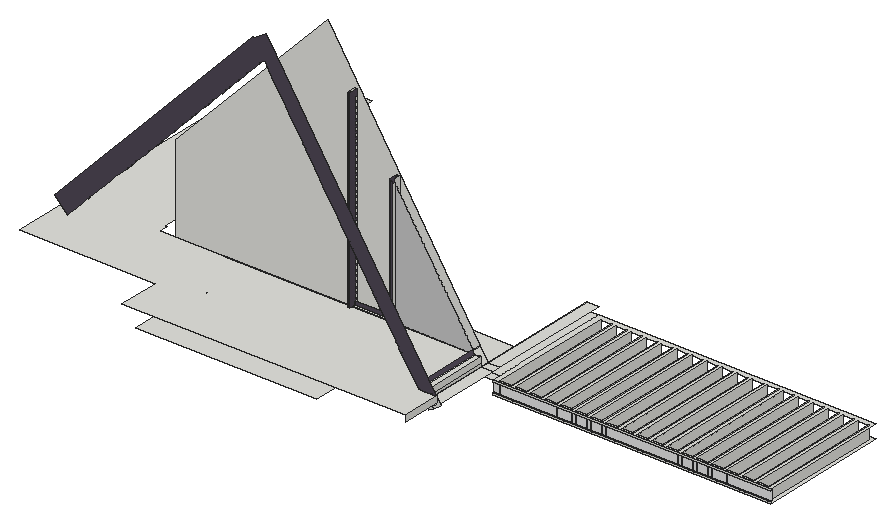
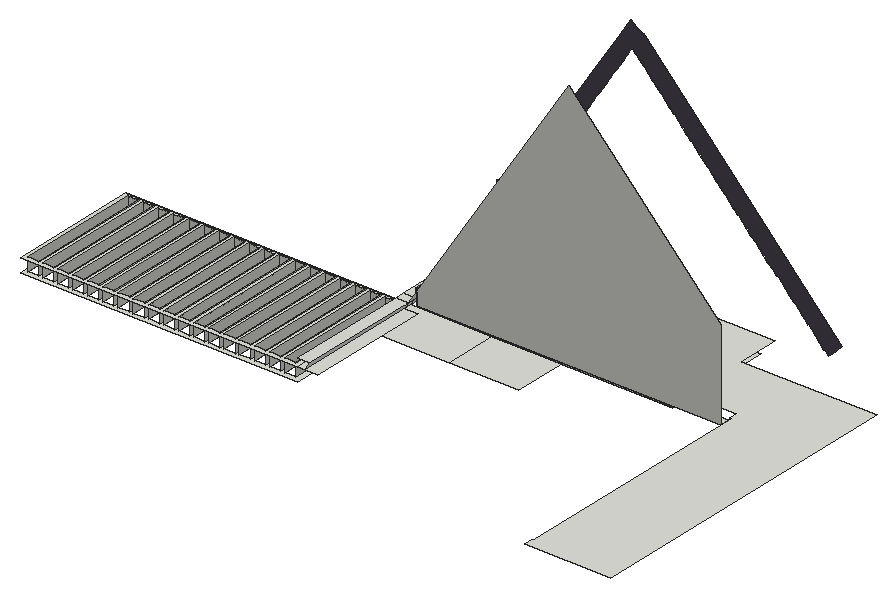
# SketchUp Ruby script. Lengths in inches.
U = 1.inch
M = Sketchup.active_model
def pt(a) = Geom::Point3d.new(a.map { |v| v * U })
def face(e, loops, mat)
  f = e.add_face(loops[0].map { |a| pt(a) })
  loops[1..].each { |l| e.add_face(l.map { |a| pt(a) }).erase! }
  f.material = f.back_material = mat if mat
  f
end
# faces: each face lists its corners as indices into pts; further lists are holes
def faces(e, pts, list, mat = nil) = list.each { |f| face(e, (f[0].is_a?(Array) ? f : [f]).map { |l| l.map { |i| pts[i] } }, mat) }
# xy, xz, yz: faces in a plane at the given z, y or x. An outline is a flat list of corners, or four numbers for a rectangle; further outlines are holes
def ring(l) = l.size == 4 ? [[l[0], l[1]], [l[2], l[1]], [l[2], l[3]], [l[0], l[3]]] : l.each_slice(2).to_a
def flat(e, list, mat, &to3) = list.each { |f| face(e, (f[0].is_a?(Array) ? f : [f]).map { |l| ring(l).map { |u, v| to3.(u, v) } }, mat) }
def xy(e, z, list, mat = nil) = flat(e, list, mat) { |x, y| [x, y, z] }
def xz(e, y, list, mat = nil) = flat(e, list, mat) { |x, z| [x, y, z] }
def yz(e, x, list, mat = nil) = flat(e, list, mat) { |y, z| [x, y, z] }
def lines(e, pts, list) = list.each { |a, b| e.add_line(pt(pts[a]), pt(pts[b])) }
# prism: a flat outline (further loops are holes) pulled along v
def prism(e, loops, v, mat = nil)
  f = face(e, loops, mat); d = Geom::Vector3d.new(v.map { |x| x * U })
  f.pushpull(f.normal.samedirection?(d) ? d.length : -d.length)
end
def box(e, o, s, mat = nil) = prism(e, [[o, [o[0] + s[0], o[1], o[2]], [o[0] + s[0], o[1] + s[1], o[2]], [o[0], o[1] + s[1], o[2]]]], [0, 0, s[2]], mat)
def at(x, y, z, deg = 0) = Geom::Transformation.translation(pt([x, y, z])) * Geom::Transformation.rotation(ORIGIN, Z_AXIS, deg.degrees)
def axes(o, x, y, z) = Geom::Transformation.new([*x, 0, *y, 0, *z, 0, *pt(o).to_a, 1])
def part(name) = M.definitions.add(name)
# library, detail: a bought-in or finely detailed component or shape, given as its bounding box
def library(name, o, s) = part(name).tap { |d| box(d.entities, o, s) }
def detail(e, o, s) = box(e.add_group.entities, o, s)
def put(e, d, t, mat = nil) = e.add_instance(d, t).tap { |i| i.material = mat if mat }
def group(e, t, mat = nil) = e.add_group.tap { |g| g.transformation = t; g.material = mat if mat }.entities
root = M.entities
M.materials.add("[Color M01]").color = [226, 226, 226]
M.materials.add("[Color M02]").color = [198, 198, 198]
M.materials.add("[Color M06]").color = [79, 71, 84]
c1 = library("A$C06767DEF\#1",[-8.3,1.21,0],[7.09,7.09,5.51])
xy(root,240.88,[[[2459.77,521.5625,2674.15,623.84],[2662.75,523.31,2671.43,620.37],[2651.06,523.31,2659.75,620.37],[2639.37,523.31,2648.06,620.37],[2627.68,523.31,2636.37,620.37],[2616,523.31,2624.68,620.37],[2604.31,523.31,2613,620.37],[2592.62,523.31,2601.31,620.37],[2580.93,523.31,2589.62,620.37],[2569.25,523.31,2577.93,620.37],[2557.56,523.31,2566.25,620.37],[2545.87,523.31,2554.56,620.37],[2534.18,523.31,2542.87,620.37],[2522.5,523.31,2531.18,620.37],[2510.81,523.31,2519.5,620.37],[2499.12,523.31,2507.81,620.37],[2487.43,523.31,2496.12,620.37],[2475.75,523.31,2484.43,620.37],[2464.06,523.31,2472.75,620.37]]])
xy(root,242.34,[[2459.77,521.5625,2674.15,522.8125]])
xy(root,249.61,[[2459.77,521.5625,2674.15,522.8125]])
xy(root,250.875,[[[2251.48,437.0625,2251.48,509.6875,2337.96,509.6875,2337.96,521.5625,2391.36,521.5625,2391.36,437.0625],[2357.39,456.39,2358.94,456.6,2360.39,457.2,2361.63,458.15,2362.59,459.39,2363.1875,460.84,2363.39,462.39,2363.1875,463.95,2362.59,465.39,2361.63,466.64,2360.39,467.59,2358.94,468.1875,2357.39,468.39,2355.84,468.1875,2354.39,467.59,2353.15,466.64,2352.19,465.39,2351.59,463.95,2351.39,462.39,2351.59,460.84,2352.19,459.39,2353.15,458.15,2354.39,457.2,2355.84,456.6],[2294.3125,459.39,2295.87,459.6,2297.3125,460.2,2298.56,461.15,2299.51,462.39,2300.11,463.84,2300.3125,465.39,2300.11,466.95,2299.51,468.39,2298.56,469.64,2297.3125,470.59,2295.87,471.1875,2294.3125,471.39,2292.76,471.1875,2291.3125,470.59,2290.07,469.64,2289.12,468.39,2288.52,466.95,2288.3125,465.39,2288.52,463.84,2289.12,462.39,2290.07,461.15,2291.3125,460.2,2292.76,459.6]]])
xy(root,251.0625,[[2251.48,509.6875,2337.96,521.5625],[2337.96,521.5625,2391.36,562.32],[2391.36,521.5625,2391.36,562.32,2444.26,562.32,2444.26,527.76,2459.77,527.76,2459.77,521.5625],[[2459.77,521.5625,2674.15,623.84],[2662.75,523.31,2671.43,620.37],[2651.06,523.31,2659.75,620.37],[2639.37,523.31,2648.06,620.37],[2627.68,523.31,2636.37,620.37],[2616,523.31,2624.68,620.37],[2604.31,523.31,2613,620.37],[2592.62,523.31,2601.31,620.37],[2580.93,523.31,2589.62,620.37],[2569.25,523.31,2577.93,620.37],[2557.56,523.31,2566.25,620.37],[2545.87,523.31,2554.56,620.37],[2534.18,523.31,2542.87,620.37],[2522.5,523.31,2531.18,620.37],[2510.81,523.31,2519.5,620.37],[2499.12,523.31,2507.81,620.37],[2487.43,523.31,2496.12,620.37],[2475.75,523.31,2484.43,620.37],[2464.06,523.31,2472.75,620.37]],[2444.26,527.76,2459.77,623.84]])
xy(root,252.25,[[2357.39,456.39,2355.84,456.6,2354.39,457.2,2353.15,458.15,2352.19,459.39,2351.59,460.84,2351.39,462.39,2351.59,463.95,2352.19,465.39,2353.15,466.64,2354.39,467.59,2355.84,468.1875,2357.39,468.39,2358.94,468.1875,2360.39,467.59,2361.63,466.64,2362.59,465.39,2363.1875,463.95,2363.39,462.39,2363.1875,460.84,2362.59,459.39,2361.63,458.15,2360.39,457.2,2358.94,456.6]])
xy(root,252.375,[[2294.3125,459.39,2292.76,459.6,2291.3125,460.2,2290.07,461.15,2289.12,462.39,2288.52,463.84,2288.3125,465.39,2288.52,466.95,2289.12,468.39,2290.07,469.64,2291.3125,470.59,2292.76,471.1875,2294.3125,471.39,2295.87,471.1875,2297.3125,470.59,2298.56,469.64,2299.51,468.39,2300.11,466.95,2300.3125,465.39,2300.11,463.84,2299.51,462.39,2298.56,461.15,2297.3125,460.2,2295.87,459.6]])
xy(root,257.0625,[[2450.46,467.1875,2459.77,521.5625],[2209.43,521.5625,2444.39,528.48],[2450.46,521.5625,2459.77,528.48],[2450.46,528.48,2459.77,623.84]])
xy(root,263.89,[[[2240.94,437.0625,2459.77,437.0625,2459.77,467.1875,2450.46,467.1875,2450.46,521.5625,2383.83,521.5625,2383.83,519.6875,2381.95,519.6875,2381.95,521.5625,2350.98,521.5625,2350.98,519.6875,2349.23,519.6875,2349.23,521.5625,2202.51,521.5625,2202.51,528.48,2200.93,528.48,2200.93,719.59,2202.51,719.59,2202.51,726.125,2135.95,726.125,2135.95,469.875,2240.94,469.875],[2203.9,480.14,2273.22,480.77]],[2349.23,519.6875,2350.98,521.5625],[2381.95,519.6875,2383.83,521.5625],[2349.23,521.5625,2350.98,526.125],[2350.98,521.5625,2381.95,523.75],
  [2381.95,521.5625,2383.83,526.125]])
xz(root,467.1875,[[2453.7,252.01,2457.75,254.61,2456.17,257.0625,2450.46,257.0625],[2457.75,254.61,2463.01,257.98,2459.77,263.03,2459.77,257.0625,2456.17,257.0625],[2450.46,257.0625,2456.17,258.95],[2456.17,257.0625,2459.77,258.95],[2450.46,258.95,2456.17,263.89],
  [2456.17,258.95,2459.77,258.95,2459.77,263.03,2459.22,263.89,2456.17,263.89],[2459.77,263.03,2459.22,263.89,2459.77,263.89]])
xz(root,467.1875,[[2450.46,257.0625,2450.46,263.89,2459.22,263.89,2335.8,456.41,2328.12,468.38,2322.86,465.01,2318.46,462.19,2317.9,462.72,2316.58,461.31,2164.37,299.61,2171.91,292.52,2175.05,289.56,2177.47,292.13,2178.35,293.0625,2180.77,295.64,2181.65,296.57,2184.07,299.14,2184.94,300.07,2187.37,302.64,2188.24,303.58,2188.02,303.79,2190.4375,306.36,2190.66,306.15,2191.54,307.08,2191.3125,307.29,2193.74,309.87,2193.96,309.65,2194.84,310.59,2197.26,313.16,2198.14,314.09,2200.56,316.66,2201.4375,317.59,2203.86,320.17,2204.74,321.1,2207.16,323.67,2208.03,324.6,2210.46,327.17,2211.33,328.11,2213.75,330.68,2214.63,331.61,2217.05,334.18,2217.93,335.11,2218.39,334.6875,2220.81,337.26,2220.35,337.6875,2221.23,338.62,2221.68,338.19,2224.11,340.76,2223.65,341.19,2224.53,342.125,2224.98,341.69,2227.4,344.27,2226.95,344.7,2227.83,345.63,2228.28,345.2,2230.7,347.77,2230.25,348.2,2231.125,349.13,2231.58,348.7,2234,351.28,2233.55,351.7,2234.42,352.64,2234.88,352.21,2237.3,354.78,2236.84,355.21,2237.72,356.14,2238.18,355.71,2240.6,358.28,2240.14,358.71,2241.02,359.64,2241.48,359.22,2243.9,361.79,2243.44,362.22,2244.32,363.15,2244.77,362.72,2247.19,365.29,2246.74,365.72,2247.62,366.65,2248.07,366.22,2250.49,368.8,2250.04,369.23,2250.92,370.16,2251.37,369.73,2253.79,372.3,2253.34,372.73,2254.21,373.66,2254.67,373.23,2257.09,375.81,2256.64,376.23,2257.51,377.17,2257.97,376.74,2260.39,379.31,2259.93,379.74,2260.8125,380.67,2261.27,380.24,2263.6875,382.8125,2263.23,383.24,2264.11,384.17,2264.56,383.75,2266.99,386.32,2266.53,386.75,2267.41,387.68,2267.86,387.25,2270.28,389.82,2269.83,390.25,2270.71,391.18,2271.16,390.75,2273.58,393.33,2273.13,393.75,2274.01,394.6875,2274.46,394.26,2276.88,396.83,2276.43,397.26,2277.3,398.19,2277.76,397.76,2280.18,400.34,2279.73,400.76,2280.6,401.7,2281.06,401.27,2283.48,403.84,2283.02,404.27,2283.9,405.2,2284.36,404.77,2286.78,407.34,2286.32,407.77,2287.2,408.7,2287.65,408.28,2290.08,410.85,2289.62,411.28,2290.5,412.21,2290.95,411.78,2293.375,414.35,2292.92,414.78,2293.8,415.71,2294.25,415.28,2296.67,417.86,2296.22,418.28,2297.1,419.22,2297.55,418.79,2299.97,421.36,2299.52,421.79,2300.39,422.72,2300.85,422.29,2303.27,424.86,2302.81,425.29,2303.69,426.23,2304.15,425.8,2306.57,428.37,2306.11,428.8,2306.99,429.73,2307.45,429.3,2309.87,431.875,2309.41,432.3,2310.29,433.23,2310.74,432.81,2313.17,435.38,2312.71,435.81,2313.59,436.74,2314.04,436.31,2316.46,438.88,2316.01,439.31,2316.89,440.24,2317.34,439.8125,2319.76,442.39,2319.31,442.8125,2320.19,443.75,2320.64,443.32,2323.0625,445.89,2322.61,446.32,2323.48,447.25,2323.9375,446.82,2326.36,449.39,2325.9,449.82,2326.17,450.11,2326.11,450.2,2326.48,450.4375,2328.05,447.99,2328.55,447.21,2328.18,446.98,2329.875,444.33,2330.24,444.57,2330.74,443.79,2330.375,443.56,2332.07,440.91,2332.4375,441.15,2332.9375,440.375,2332.57,440.14,2334.26,437.49,2334.63,437.73,2335.13,436.95,2334.76,436.72,2336.45,434.07,2336.82,434.31,2337.32,433.53,2336.95,433.3,2338.65,430.65,2339.02,430.89,2339.51,430.11,2339.14,429.88,2340.84,427.23,2341.21,427.47,2341.71,426.69,2341.34,426.46,2343.03,423.8125,2343.4,424.05,2343.9,423.27,2343.53,423.04,2345.22,420.39,2345.59,420.63,2346.09,419.85,2345.72,419.62,2347.42,416.97,2347.79,417.21,2348.28,416.43,2347.92,416.2,2349.61,413.55,2349.98,413.79,2350.48,413.01,2350.11,412.78,2351.8,410.13,2352.17,410.37,2352.67,409.59,2352.3,409.36,2354,406.71,2354.36,406.95,2354.86,406.17,2354.49,405.9375,2356.1875,403.29,2356.56,403.53,2357.05,402.75,2356.6875,402.52,2358.38,399.875,2358.75,400.11,2359.25,399.33,2358.88,399.1,2360.57,396.45,2360.94,396.69,2361.4375,395.91,2361.07,395.68,2362.77,393.03,2363.13,393.27,2363.63,392.49,2363.26,392.26,2364.96,389.61,2365.33,389.85,2365.82,389.07,2365.46,388.84,2367.15,386.19,2367.52,386.43,2368.02,385.65,2367.65,385.42,2369.34,382.77,2369.71,383.01,2370.21,382.23,2369.84,382,2371.54,379.35,2371.9,379.59,2372.4,378.8125,2372.03,378.58,2373.73,375.93,2374.1,376.17,2374.59,375.39,2374.23,375.16,2375.92,372.51,2376.29,372.75,2376.79,371.97,2376.42,371.74,2378.11,369.09,2378.48,369.33,2379.11,368.34,2378.75,368.11,2380.44,365.46,2380.81,365.7,2381.44,364.71,2383.14,362.07,2383.77,361.08,2383.4,360.85,2385.1,358.2,2385.46,358.4375,2386.1,357.45,2385.73,357.22,2387.42,354.57,2387.79,354.81,2388.43,353.82,2388.06,353.58,2389.75,350.94,2390.12,351.18,2390.75,350.19,2390.38,349.95,2392.08,347.3125,2392.45,347.55,2393.08,346.56,2392.71,346.32,2394.41,343.68,2394.77,343.92,2395.41,342.93,2395.04,342.69,2396.73,340.05,2397.1,340.29,2397.63,339.46,2397.27,339.22,2398.96,336.58,2399.33,336.8125,2399.86,335.98,2399.49,335.75,2401.1875,333.11,2401.55,333.34,2402.09,332.51,2401.72,332.28,2403.41,329.63,2403.78,329.87,2404.3125,329.04,2403.94,328.8,2405.64,326.16,2406.01,326.4,2406.54,325.57,2406.17,325.33,2407.87,322.6875,2408.23,322.92,2408.77,322.09,2408.4,321.86,2410.09,319.21,2410.46,319.45,2410.99,318.62,2410.625,318.38,2412.32,315.74,2412.6875,315.98,2413.22,315.15,2412.85,314.91,2414.54,312.27,2414.91,312.51,2415.44,311.68,2415.08,311.44,2416.77,308.8,2417.14,309.03,2417.67,308.2,2417.3,307.97,2419,305.32,2419.37,305.56,2419.9,304.73,2419.53,304.49,2421.22,301.85,2421.59,302.09,2422.125,301.26,2421.86,301.09,2423.55,298.45,2423.82,298.61,2424.35,297.79,2424.09,297.62,2425.78,294.97,2426.04,295.14,2426.58,294.3125,2426.3125,294.14,2428.01,291.5,2428.27,291.67,2428.8,290.84,2428.54,290.67,2430.23,288.03,2430.5,288.2,2431.03,287.37,2430.77,287.2,2432.46,284.56,2432.72,284.72,2433.26,283.89,2432.99,283.73,2434.6875,281.08,2434.95,281.25,2435.48,280.42,2435.22,280.25,2436.91,277.61,2437.18,277.78,2437.71,276.95,2437.44,276.78,2439.14,274.14,2439.4,274.31,2439.93,273.48,2439.67,273.31,2441.37,270.67,2441.63,270.83,2442.16,270,2441.9,269.84,2443.59,267.19,2443.86,267.36,2444.39,266.53,2444.125,266.36,2445.82,263.72,2446.08,263.89]],"[Color M06]")
xz(root,509.6875,[[2251.48,250.875,2337.96,251.0625]])
xz(root,519.6875,[[2349.23,263.89,2350.98,412.22],[2381.95,263.89,2383.83,263.89,2383.83,360.99,2383.46,360.76,2383.4,360.85,2383.77,361.08,2383.14,362.07,2382.77,361.83,2381.95,363.11]],"[Color M06]")
xz(root,521.5625,[[2459.77,240.88,2674.15,242.34],[2459.77,249.61,2674.15,251.0625],[2337.96,250.875,2391.36,251.0625],[2251.48,251.0625,2391.36,257.0625],[2251.48,257.0625,2391.36,258.95],
  [2391.36,257.0625,2444.39,258.95],[2444.39,257.0625,2450.46,257.0625,2449.25,258.95,2444.39,258.95],[2450.46,257.0625,2449.25,258.95,2450.46,258.95],[2251.48,258.95,2391.36,263.89],[2391.36,258.95,2444.39,263.89],
  [2444.39,258.95,2449.25,258.95,2446.08,263.89,2445.82,263.72,2445.71,263.89,2444.39,263.89],[2449.25,258.95,2446.08,263.89,2449.25,263.89],[2449.25,258.95,2450.46,263.89],[2445.82,263.72,2445.71,263.89,2446.08,263.89],[2444.39,263.89,2445.71,263.89,2444.39,265.95],
  [2445.71,263.89,2446.08,263.89,2444.39,266.53,2444.39,265.95]])
xz(root,521.5625,[[2383.83,263.89,2444.39,263.89,2444.39,265.95,2444.125,266.36,2444.39,266.53,2443.86,267.36,2443.59,267.19,2441.9,269.84,2442.16,270,2441.63,270.83,2441.37,270.67,2439.67,273.31,2439.93,273.48,2439.4,274.31,2439.14,274.14,2437.44,276.78,2437.71,276.95,2437.18,277.78,2436.91,277.61,2435.22,280.25,2435.48,280.42,2434.95,281.25,2434.6875,281.08,2432.99,283.73,2433.26,283.89,2432.72,284.72,2432.46,284.56,2430.77,287.2,2431.03,287.37,2430.5,288.2,2430.23,288.03,2428.54,290.67,2428.8,290.84,2428.27,291.67,2428.01,291.5,2426.3125,294.14,2426.58,294.3125,2426.04,295.14,2425.78,294.97,2424.09,297.62,2424.35,297.79,2423.82,298.61,2423.55,298.45,2421.86,301.09,2422.125,301.26,2421.59,302.09,2421.22,301.85,2419.53,304.49,2419.9,304.73,2419.37,305.56,2419,305.32,2417.3,307.97,2417.67,308.2,2417.14,309.03,2416.77,308.8,2415.08,311.44,2415.44,311.68,2414.91,312.51,2414.54,312.27,2412.85,314.91,2413.22,315.15,2412.6875,315.98,2412.32,315.74,2410.625,318.38,2410.99,318.62,2410.46,319.45,2410.09,319.21,2408.4,321.86,2408.77,322.09,2408.23,322.92,2407.87,322.6875,2406.17,325.33,2406.54,325.57,2406.01,326.4,2405.64,326.16,2403.94,328.8,2404.3125,329.04,2403.78,329.87,2403.41,329.63,2401.72,332.28,2402.09,332.51,2401.55,333.34,2401.1875,333.11,2399.49,335.75,2399.86,335.98,2399.33,336.8125,2398.96,336.58,2397.27,339.22,2397.63,339.46,2397.21,340.125,2397.1,340.29,2396.73,340.05,2395.04,342.69,2395.41,342.93,2394.77,343.92,2394.41,343.68,2392.71,346.32,2393.08,346.56,2392.45,347.55,2392.08,347.3125,2390.38,349.95,2390.75,350.19,2390.12,351.18,2389.75,350.94,2388.06,353.58,2388.43,353.82,2387.79,354.81,2387.42,354.57,2385.73,357.22,2386.1,357.45,2385.46,358.4375,2385.1,358.2,2383.83,360.18]],"[Color M02]")
xz(root,522.8125,[[2459.77,242.34,2674.15,249.61]],"[Color M01]")
xz(root,523.31,[[2464.06,240.88,2472.75,251.0625],[2475.75,240.88,2484.43,251.0625],[2487.43,240.88,2496.12,251.0625],[2499.12,240.88,2507.81,251.0625],[2510.81,240.88,2519.5,251.0625],
  [2522.5,240.88,2531.18,251.0625],[2534.18,240.88,2542.87,251.0625],[2545.87,240.88,2554.56,251.0625],[2557.56,240.88,2566.25,251.0625],[2569.25,240.88,2577.93,251.0625],
  [2580.93,240.88,2589.62,251.0625],[2592.62,240.88,2601.31,251.0625],[2604.31,240.88,2613,251.0625],[2616,240.88,2624.68,251.0625],[2627.68,240.88,2636.37,251.0625],
  [2639.37,240.88,2648.06,251.0625],[2651.06,240.88,2659.75,251.0625],[2662.75,240.88,2671.43,251.0625]])
xz(root,523.75,[[2350.98,263.89,2381.95,267.02]],"[Color M06]")
xz(root,526.125,[[2349.23,263.89,2350.98,412.22],[2381.95,263.89,2383.83,363.92]])
xz(root,528.48,[[2209.43,257.0625,2209.43,326.08,2326.48,450.4375,2444.39,266.53,2444.39,257.0625]])
yz(root,2337.96,[[509.6875,250.875,521.5625,251.0625]])
yz(root,2349.23,[[521.5625,263.89,526.125,412.22]])
yz(root,2349.23,[[519.6875,263.89,521.5625,412.22]],"[Color M06]")
yz(root,2350.98,[[523.75,263.89,526.125,267.02]])
yz(root,2350.98,[[519.6875,263.89,523.75,263.89,523.75,267.02,526.125,267.02,526.125,267.83,523.75,267.83,523.75,270.95,526.125,270.95,526.125,271.76,523.75,271.76,523.75,274.89,526.125,274.89,526.125,275.7,523.75,275.7,523.75,278.83,526.125,278.83,526.125,279.64,523.75,279.64,523.75,282.77,526.125,282.77,526.125,283.58,523.75,283.58,523.75,286.7,526.125,286.7,526.125,287.51,523.75,287.51,523.75,290.64,526.125,290.64,526.125,291.45,523.75,291.45,523.75,294.58,526.125,294.58,526.125,295.39,523.75,295.39,523.75,298.52,526.125,298.52,526.125,299.33,523.75,299.33,523.75,302.45,526.125,302.45,526.125,303.26,523.75,303.26,523.75,306.39,526.125,306.39,526.125,307.2,523.75,307.2,523.75,310.33,526.125,310.33,526.125,311.14,523.75,311.14,523.75,314.27,526.125,314.27,526.125,315.08,524.25,315.08,524.25,318.2,526.125,318.2,526.125,319.01,524.25,319.01,524.25,322.14,526.125,322.14,526.125,322.89,524.25,322.89,524.25,326.02,526.125,326.02,526.125,326.76,524.25,326.76,524.25,329.89,526.125,329.89,526.125,330.64,524.25,330.64,524.25,333.77,526.125,333.77,526.125,334.51,524.25,334.51,524.25,337.64,526.125,337.64,526.125,338.39,524.25,338.39,524.25,341.52,526.125,341.52,526.125,341.93,524.25,341.93,524.25,345.06,526.125,345.06,526.125,346,524.25,346,524.25,349.12,526.125,349.12,526.125,350.06,524.25,350.06,524.25,353.18,526.125,353.18,526.125,354.12,524.25,354.12,524.25,357.25,526.125,357.25,526.125,358.06,524.25,358.06,524.25,361.18,526.125,361.18,526.125,362,524.25,362,524.25,365.12,526.125,365.12,526.125,366.25,524.25,366.25,524.25,369.37,526.125,369.37,526.125,370.5,524.25,370.5,524.25,373.62,526.125,373.62,526.125,374.75,524.25,374.75,524.25,377.87,526.125,377.87,526.125,379,524.25,379,524.25,382.12,526.125,382.12,526.125,383.25,524.25,383.25,524.25,386.37,526.125,386.37,526.125,387.5,524.25,387.5,524.25,390.62,526.125,390.62,526.125,391.75,524.25,391.75,524.25,394.87,526.125,394.87,526.125,396,524.25,396,524.25,399.12,526.125,399.12,526.125,400.25,524.25,400.25,524.25,403.37,526.125,403.37,526.125,404.5,524.25,404.5,524.25,407.62,526.125,407.62,526.125,412.22,519.6875,412.22]],"[Color M06]")
yz(root,2381.95,[[523.75,263.89,526.125,267.02]])
yz(root,2381.95,[[519.6875,263.89,519.6875,363.92,524.25,363.92,524.25,362,526.125,362,526.125,361.18,524.25,361.18,524.25,358.06,526.125,358.06,526.125,357.25,524.25,357.25,524.25,354.12,526.125,354.12,526.125,353.18,524.25,353.18,524.25,350.06,526.125,350.06,526.125,349.12,524.25,349.12,524.25,346,526.125,346,526.125,345.06,524.25,345.06,524.25,341.93,526.125,341.93,526.125,341.52,524.25,341.52,524.25,338.39,526.125,338.39,526.125,337.64,524.25,337.64,524.25,334.51,526.125,334.51,526.125,333.77,524.25,333.77,524.25,330.64,526.125,330.64,526.125,329.89,524.25,329.89,524.25,326.76,526.125,326.76,526.125,326.02,524.25,326.02,524.25,322.89,526.125,322.89,526.125,322.14,524.25,322.14,524.25,319.01,526.125,319.01,526.125,318.2,524.25,318.2,524.25,315.08,526.125,315.08,526.125,314.27,523.75,314.27,523.75,311.14,526.125,311.14,526.125,310.33,523.75,310.33,523.75,307.2,526.125,307.2,526.125,306.39,523.75,306.39,523.75,303.26,526.125,303.26,526.125,302.45,523.75,302.45,523.75,299.33,526.125,299.33,526.125,298.52,523.75,298.52,523.75,295.39,526.125,295.39,526.125,294.58,523.75,294.58,523.75,291.45,526.125,291.45,526.125,290.64,523.75,290.64,523.75,287.51,526.125,287.51,526.125,286.7,523.75,286.7,523.75,283.58,526.125,283.58,526.125,282.77,523.75,282.77,523.75,279.64,526.125,279.64,526.125,278.83,523.75,278.83,523.75,275.7,526.125,275.7,526.125,274.89,523.75,274.89,523.75,271.76,526.125,271.76,526.125,270.95,523.75,270.95,523.75,267.83,526.125,267.83,526.125,267.02,523.75,267.02,523.75,263.89]],"[Color M06]")
yz(root,2383.83,[[519.6875,263.89,521.5625,360.99],[521.5625,263.89,526.125,363.92]])
yz(root,2444.39,[[521.5625,257.0625,528.48,266.53]])
yz(root,2450.46,[[467.1875,257.0625,521.5625,258.95],[467.1875,258.95,521.5625,263.89]])
yz(root,2459.77,[[437.0625,258.95,467.1875,263.89]])
yz(root,2464.06,[[523.31,240.88,620.37,251.0625]])
yz(root,2472.75,[[523.31,240.88,620.37,251.0625]])
yz(root,2475.75,[[523.31,240.88,620.37,251.0625]])
yz(root,2484.43,[[523.31,240.88,620.37,251.0625]])
yz(root,2487.43,[[523.31,240.88,620.37,251.0625]])
yz(root,2496.12,[[523.31,240.88,620.37,251.0625]])
yz(root,2499.12,[[523.31,240.88,620.37,251.0625]])
yz(root,2507.81,[[523.31,240.88,620.37,251.0625]])
yz(root,2510.81,[[523.31,240.88,620.37,251.0625]])
yz(root,2519.5,[[523.31,240.88,620.37,251.0625]])
yz(root,2522.5,[[523.31,240.88,620.37,251.0625]])
yz(root,2531.18,[[523.31,240.88,620.37,251.0625]])
yz(root,2534.18,[[523.31,240.88,620.37,251.0625]])
yz(root,2542.87,[[523.31,240.88,620.37,251.0625]])
yz(root,2545.87,[[523.31,240.88,620.37,251.0625]])
yz(root,2554.56,[[523.31,240.88,620.37,251.0625]])
yz(root,2557.56,[[523.31,240.88,620.37,251.0625]])
yz(root,2566.25,[[523.31,240.88,620.37,251.0625]])
yz(root,2569.25,[[523.31,240.88,620.37,251.0625]])
yz(root,2577.93,[[523.31,240.88,620.37,251.0625]])
yz(root,2580.93,[[523.31,240.88,620.37,251.0625]])
yz(root,2589.62,[[523.31,240.88,620.37,251.0625]])
yz(root,2592.62,[[523.31,240.88,620.37,251.0625]])
yz(root,2601.31,[[523.31,240.88,620.37,251.0625]])
yz(root,2604.31,[[523.31,240.88,620.37,251.0625]])
yz(root,2613,[[523.31,240.88,620.37,251.0625]])
yz(root,2616,[[523.31,240.88,620.37,251.0625]])
yz(root,2624.68,[[523.31,240.88,620.37,251.0625]])
yz(root,2627.68,[[523.31,240.88,620.37,251.0625]])
yz(root,2636.37,[[523.31,240.88,620.37,251.0625]])
yz(root,2639.37,[[523.31,240.88,620.37,251.0625]])
yz(root,2648.06,[[523.31,240.88,620.37,251.0625]])
yz(root,2651.06,[[523.31,240.88,620.37,251.0625]])
yz(root,2659.75,[[523.31,240.88,620.37,251.0625]])
yz(root,2662.75,[[523.31,240.88,620.37,251.0625]])
yz(root,2671.43,[[523.31,240.88,620.37,251.0625]])
p = [[2357.39,456.39,250.875],[2355.84,456.6,250.875],[2355.84,456.6,252.25],[2357.39,456.39,252.25],[2358.94,456.6,250.875],[2358.94,456.6,252.25],
  [2354.39,457.2,250.875],[2354.39,457.2,252.25],[2360.39,457.2,250.875],[2360.39,457.2,252.25],[2353.15,458.15,250.875],[2353.15,458.15,252.25],
  [2361.63,458.15,250.875],[2361.63,458.15,252.25],[2352.19,459.39,250.875],[2352.19,459.39,252.25],[2362.59,459.39,250.875],[2362.59,459.39,252.25],
  [2294.3125,459.39,250.875],[2292.76,459.6,250.875],[2292.76,459.6,252.375],[2294.3125,459.39,252.375],[2295.87,459.6,250.875],[2295.87,459.6,252.375],
  [2351.59,460.84,250.875],[2351.59,460.84,252.25],[2363.1875,460.84,250.875],[2363.1875,460.84,252.25],[2291.3125,460.2,250.875],[2291.3125,460.2,252.375],
  [2297.3125,460.2,250.875],[2297.3125,460.2,252.375],[2290.07,461.15,250.875],[2290.07,461.15,252.375],[2298.56,461.15,250.875],[2298.56,461.15,252.375],
  [2351.39,462.39,250.875],[2351.39,462.39,252.25],[2363.39,462.39,250.875],[2363.39,462.39,252.25],[2289.12,462.39,250.875],[2289.12,462.39,252.375],
  [2299.51,462.39,250.875],[2299.51,462.39,252.375],[2288.52,463.84,250.875],[2288.52,463.84,252.375],[2300.11,463.84,250.875],[2300.11,463.84,252.375],
  [2351.59,463.95,250.875],[2351.59,463.95,252.25],[2363.1875,463.95,250.875],[2363.1875,463.95,252.25],[2300.3125,465.39,250.875],[2300.3125,465.39,252.375],
  [2352.19,465.39,250.875],[2352.19,465.39,252.25],[2362.59,465.39,250.875],[2362.59,465.39,252.25],[2300.11,466.95,250.875],[2300.11,466.95,252.375],
  [2353.15,466.64,250.875],[2353.15,466.64,252.25],[2361.63,466.64,250.875],[2361.63,466.64,252.25],[2354.39,467.59,250.875],[2354.39,467.59,252.25],
  [2360.39,467.59,250.875],[2360.39,467.59,252.25],[2288.52,466.95,250.875],[2289.12,468.39,250.875],[2289.12,468.39,252.375],[2288.52,466.95,252.375],
  [2299.51,468.39,250.875],[2299.51,468.39,252.375],[2355.84,468.1875,250.875],[2355.84,468.1875,252.25],[2358.94,468.1875,250.875],[2358.94,468.1875,252.25],
  [2357.39,468.39,250.875],[2357.39,468.39,252.25],[2290.07,469.64,250.875],[2290.07,469.64,252.375],[2298.56,469.64,250.875],[2298.56,469.64,252.375],
  [2291.3125,470.59,250.875],[2291.3125,470.59,252.375],[2297.3125,470.59,250.875],[2297.3125,470.59,252.375],[2292.76,471.1875,250.875],[2292.76,471.1875,252.375],
  [2295.87,471.1875,250.875],[2295.87,471.1875,252.375],[2294.3125,471.39,250.875],[2294.3125,471.39,252.375],[2450.46,467.1875,257.0625],[2450.46,521.5625,257.0625],
  [2453.7,521.5625,252.01],[2453.7,467.1875,252.01],[2450.46,528.48,257.0625],[2453.7,528.48,252.01],[2450.46,623.84,257.0625],[2453.7,623.84,252.01],
  [2446.08,467.1875,263.89],[2446.08,521.5625,263.89],[2449.25,521.5625,258.95],[2444.39,528.48,266.53],[2444.39,521.5625,266.53],[2444.125,521.5625,266.36],
  [2444.39,521.5625,265.95],[2445.71,521.5625,263.89],[2445.82,521.5625,263.72],[2445.82,467.1875,263.72],[2444.125,467.1875,266.36]]
faces(root,p,[[0,1,2,3],[4,0,3,5],[1,6,7,2],[8,4,5,9],[6,10,11,7],[12,8,9,13],[10,14,15,11],[16,12,13,17],
  [18,19,20,21],[22,18,21,23],[14,24,25,15],[26,16,17,27],[19,28,29,20],[30,22,23,31],[28,32,33,29],[34,30,31,35],
  [24,36,37,25],[38,26,27,39],[32,40,41,33],[42,34,35,43],[40,44,45,41],[46,42,43,47],[36,48,49,37],[50,38,39,51],
  [52,46,47,53],[48,54,55,49],[56,50,51,57],[58,52,53,59],[54,60,61,55],[62,56,57,63],[60,64,65,61],[66,62,63,67],
  [68,69,70,71],[72,58,59,73],[64,74,75,65],[76,66,67,77],[74,78,79,75],[78,76,77,79],[69,80,81,70],[82,72,73,83],
  [80,84,85,81],[86,82,83,87],[84,88,89,85],[90,86,87,91],[88,92,93,89],[92,90,91,93],[94,95,96,97],[95,98,99,96],
  [98,100,101,99],[94,102,103,104,95],[98,105,106,103,104,95],[103,102,111,110]])
faces(root,p,[[107,108,109,110,111,112]],"[Color M06]")
put(root,c1,axes([2299.92,464.17,249.52],[1.14885,0,0],[0,0.84644,0],[0,0,0.5175]))
put(root,c1,axes([2363.98,458.37,248.02],[1.14885,0,0],[0,0.84644,0],[0,0,0.5175]))
